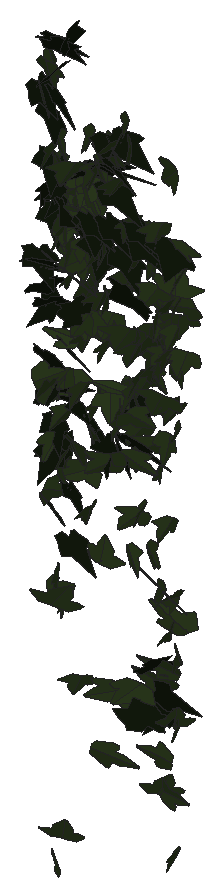
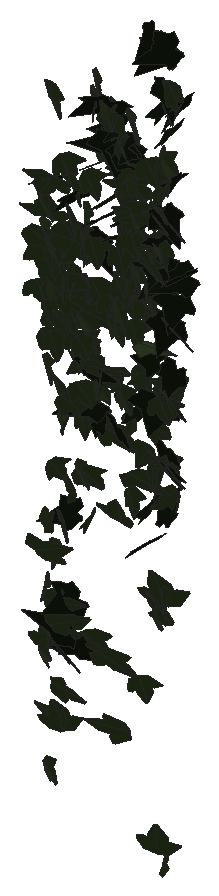
# SketchUp Ruby script. Lengths in millimetres.
U = 1.mm
M = Sketchup.active_model
def pt(a) = Geom::Point3d.new(a.map { |v| v * U })
def face(e, loops, mat)
  f = e.add_face(loops[0].map { |a| pt(a) })
  loops[1..].each { |l| e.add_face(l.map { |a| pt(a) }).erase! }
  f.material = f.back_material = mat if mat
  f
end
# faces: each face lists its corners as indices into pts; further lists are holes
def faces(e, pts, list, mat = nil) = list.each { |f| face(e, (f[0].is_a?(Array) ? f : [f]).map { |l| l.map { |i| pts[i] } }, mat) }
# xy, xz, yz: faces in a plane at the given z, y or x. An outline is a flat list of corners, or four numbers for a rectangle; further outlines are holes
def ring(l) = l.size == 4 ? [[l[0], l[1]], [l[2], l[1]], [l[2], l[3]], [l[0], l[3]]] : l.each_slice(2).to_a
def flat(e, list, mat, &to3) = list.each { |f| face(e, (f[0].is_a?(Array) ? f : [f]).map { |l| ring(l).map { |u, v| to3.(u, v) } }, mat) }
def xy(e, z, list, mat = nil) = flat(e, list, mat) { |x, y| [x, y, z] }
def xz(e, y, list, mat = nil) = flat(e, list, mat) { |x, z| [x, y, z] }
def yz(e, x, list, mat = nil) = flat(e, list, mat) { |y, z| [x, y, z] }
def lines(e, pts, list) = list.each { |a, b| e.add_line(pt(pts[a]), pt(pts[b])) }
# prism: a flat outline (further loops are holes) pulled along v
def prism(e, loops, v, mat = nil)
  f = face(e, loops, mat); d = Geom::Vector3d.new(v.map { |x| x * U })
  f.pushpull(f.normal.samedirection?(d) ? d.length : -d.length)
end
def box(e, o, s, mat = nil) = prism(e, [[o, [o[0] + s[0], o[1], o[2]], [o[0] + s[0], o[1] + s[1], o[2]], [o[0], o[1] + s[1], o[2]]]], [0, 0, s[2]], mat)
def at(x, y, z, deg = 0) = Geom::Transformation.translation(pt([x, y, z])) * Geom::Transformation.rotation(ORIGIN, Z_AXIS, deg.degrees)
def axes(o, x, y, z) = Geom::Transformation.new([*x, 0, *y, 0, *z, 0, *pt(o).to_a, 1])
def part(name) = M.definitions.add(name)
# library, detail: a bought-in or finely detailed component or shape, given as its bounding box
def library(name, o, s) = part(name).tap { |d| box(d.entities, o, s) }
def detail(e, o, s) = box(e.add_group.entities, o, s)
def put(e, d, t, mat = nil) = e.add_instance(d, t).tap { |i| i.material = mat if mat }
def group(e, t, mat = nil) = e.add_group.tap { |g| g.transformation = t; g.material = mat if mat }.entities
root = M.entities
M.materials.add("efeu1").color = [18, 25, 13]
M.materials.add("efeu2").color = [43, 57, 29]
c1 = part("ivyleaf_9")
p = [[39.1,54.8,31.7],[34.5,51.8,30.2],[-5.3,25.2,17.3],[-17.9,28.3,20.9],[-21.6,21.7,17],[-20.2,4.3,5.3],
  [-22.9,-0.3,2.5],[-17.1,-4,-0.6],[-2,-2.1,-1.2],[-0.7,-15.4,-10.1],[16.6,-22.3,-16.7],[21.1,-15.1,-12.5],
  [32.7,-10.7,-11],[46.1,-1.8,-6.6],[30.8,11.2,3.8]]
faces(c1.entities,p,[[0,1,2,3,4,5,6,7,8,9,10,11,12,13,14]],"efeu1")
c2 = part("ivyleaf_10")
p = [[0,12.8,-0.8],[-1.5,51.3,-10.9],[-4.9,51,-11.6],[-13.6,26.5,-7.3],[-13.2,15.9,-4.6],[-21.1,19.3,-7.2],
  [-29.5,16.3,-8.3],[-29.2,8.3,-6.2],[-19.7,-9.8,0.5],[-7.6,-13,4],[1,-12.2,5.8],[-0.4,51.1,-11.1],
  [-1.5,51.1,-10.9],[1,-12.4,5.9],[16.9,-12.4,3.5],[35.1,9.1,-5.1],[35,12.9,-6.1],[20.5,16.4,-4.9],
  [15.8,15,-3.8],[15.3,27.6,-7.1],[12.8,31.3,-7.8]]
faces(c2.entities,p,[[0,1,2,3,4,5,6,7,8,9,10],[11,12,0,13,14,15,16,17,18,19,20]],"efeu2")
put(root,c1,axes([810.5,996.7,1201],[0.11506,-0.81585,-0.18626],[0.13224,0.19777,-0.81138],[1.01235,0.06689,0.12716]))
put(root,c1,axes([829,1016.4,1320.9],[0.0026,0.65958,-0.47998],[0.00539,-0.47998,-0.65957],[-0.99518,-0.00087,-0.00482]))
put(root,c1,axes([825,987,1153.9],[0.42912,0.77528,0.01543],[-0.03301,0.0292,-0.85055],[-0.94545,0.35086,0.0367]))
put(root,c1,axes([834.5,1004,1112.6],[-0.90751,0.29825,-0.1157],[0.10865,-0.08822,-0.79997],[-0.37486,-0.74762,0.04824]))
put(root,c2,axes([829.4,1024.7,975],[-0.67201,-0.58372,0.16905],[-0.05048,-0.18053,-0.67875],[1.1555,-0.34737,0.06866]))
put(root,c1,axes([810.7,979.3,1192.1],[0.97056,0.14562,0.3072],[0.30233,0.2868,-0.77769],[-0.28395,0.80312,0.22202]))
put(root,c2,axes([813.2,1019.4,1543.2],[0.66337,-0.38918,0.43163],[0.57841,-0.04483,-0.63768],[0.41008,0.69279,0.20121]))
put(root,c1,axes([822.5,996.2,1025],[0.90634,0.10167,-0.35465],[-0.43015,-0.03911,-0.74979],[-0.13252,0.82229,0.00819]))
put(root,c1,axes([823.6,1004.6,1115],[0.72058,0.53904,-0.10921],[-0.11452,-0.0591,-0.7994],[-0.66114,0.59774,0.01944]))
put(root,c2,axes([827.9,999.2,1539.6],[-0.93809,0.19423,-0.00204],[0.00246,-0.00033,-0.79308],[-0.23696,-0.76893,-0.00017]))
put(root,c1,axes([819.5,985,1509.9],[0.38084,-0.64426,-0.50578],[-0.29332,0.44535,-0.71567],[0.95525,0.3936,-0.01811]))
put(root,c1,axes([840.7,1016.9,1320.5],[-0.80703,0.43923,0.04747],[-0.05481,0.01816,-0.79398],[-0.53618,-0.66295,0.00971]))
put(root,c2,axes([824.1,1024.8,623.6],[0.38639,-0.70982,0.08083],[0.19588,-0.01543,-0.76463],[0.84928,0.3265,0.13958]))
put(root,c2,axes([829.5,1012,866.3],[0.65073,0.43394,-0.30362],[-0.28178,-0.19718,-0.68757],[-0.58144,0.58121,-0.00658]))
put(root,c2,axes([824.3,989.7,1500.2],[-0.30724,0.76906,-0.17946],[0.02498,-0.18053,-0.78547],[-1.50279,-0.16023,0.02363]))
put(root,c2,axes([830,1011.9,1374],[-0.74422,0.53273,0.01084],[-0.0148,0.00259,-0.80987],[-0.6499,-0.61011,0.00602]))
put(root,c1,axes([831.1,985.7,952],[-0.64911,0.64885,0.05088],[0.02724,-0.04748,0.839],[0.79356,0.53237,0.01282]))
put(root,c1,axes([822,1021.8,893.4],[-0.5232,-0.16914,-0.62901],[0.75846,0.1184,-0.4557],[0.23709,-0.75203,0.06972]))
put(root,c1,axes([834.2,1005.5,849.9],[-0.87825,-0.08211,-0.33222],[0.4085,-0.00923,-0.72328],[0.08621,-0.79279,0.04282]))
put(root,c2,axes([820.4,1017.4,978.1],[0.70979,-0.24084,0.46021],[0.54301,-0.12506,-0.62813],[0.32666,0.73119,0.04415]))
put(root,c1,axes([842.1,990.6,1533.2],[-0.08532,0.8345,0.0914],[-0.02687,0.08986,-0.8373],[-1.02382,-0.0719,0.01435]))
put(root,c1,axes([829.3,1008.1,1370.5],[-0.10934,-0.82441,0.06829],[-0.02446,-0.0665,-0.82917],[1.00893,-0.09096,-0.0127]))
put(root,c1,axes([853.1,1011.4,860.7],[-0.85867,0.37249,0.21429],[-0.22636,0.10751,-0.79628],[-0.47289,-0.72783,-0.00795]))
put(root,c1,axes([844.2,1018.4,1307.9],[-0.86231,0.26897,-0.29214],[0.30251,-0.16693,-0.75361],[-0.37841,-0.74637,0.06327]))
put(root,c2,axes([819,1026.4,587],[0.82164,-0.31501,-0.50248],[0.7449,-0.3156,0.53413],[-0.84799,-0.58245,-0.01767]))
put(root,c2,axes([839.3,1020.9,159],[-1.16169,-0.28412,0.00304],[0.02764,-0.024,0.6727],[-0.54007,0.60992,0.02788]))
put(root,c2,axes([838.7,998.5,1399.6],[0.28935,-0.66536,0.39424],[0.15419,-0.38587,-0.68248],[1.46381,0.17217,-0.00604]))
put(root,c2,axes([841.8,1009.1,1256.9],[0.93948,-0.49893,-0.30782],[-0.14501,0.3444,-0.6804],[1.10628,0.46884,0.17223]))
put(root,c2,axes([846.7,1003.9,826.1],[-0.28859,0.32204,0.73224],[-0.49041,0.61231,-0.39915],[-0.84374,-0.46605,-0.01845]))
put(root,c1,axes([835.5,1019.9,1271.6],[-0.44811,-0.67676,-0.18819],[0.16019,0.14248,-0.76863],[0.84187,-0.38734,0.04608]))
put(root,c2,axes([837.7,1011.4,1365.1],[-0.22319,0.76666,0.10713],[-0.00851,0.10844,-0.78797],[-0.94437,-0.18217,-0.01822]))
put(root,c2,axes([842,1003.2,111.6],[-0.55913,0.52209,0.12956],[0.09511,-0.10394,0.69464],[0.64934,0.46478,0.00981]))
put(root,c2,axes([837.8,975.5,965],[0.10638,-0.45049,0.76235],[-0.04277,0.76368,0.45529],[-1.07946,-0.07465,0.05709]))
put(root,c1,axes([839.5,999.9,747.9],[0.61069,-0.60501,0.06345],[-0.02629,0.06448,0.78486],[-0.74169,-0.50043,0.02442]))
put(root,c1,axes([830.2,1003.1,1454],[0.09681,-0.75562,0.34801],[0.13592,-0.33679,-0.75665],[1.00578,0.11824,0.06876]))
put(root,c2,axes([836.1,988.1,790.7],[-0.17922,-0.3112,-0.73197],[0.44016,0.6373,-0.34335],[0.86479,-0.38886,0.02307]))
put(root,c2,axes([833,995.9,976.6],[0.23446,0.47738,0.64728],[0.26902,0.60873,-0.51442],[-0.94362,0.29216,0.01417]))
put(root,c2,axes([828.7,979,989.3],[0.21438,0.13816,-0.8179],[0.76135,0.52876,0.22339],[0.66667,-0.64827,0.00789]))
put(root,c2,axes([846.1,1017.2,920.3],[-0.11888,-0.46927,0.50324],[0.08472,-0.50701,-0.46726],[1.30683,-0.00982,0.07607]))
put(root,c2,axes([843,1005.7,1416.2],[-0.37776,0.74695,0.02492],[-0.00674,0.02469,-0.80857],[-0.91176,-0.30966,-0.00435]))
put(root,c2,axes([842.6,1019,1321.3],[0.82884,-0.38508,0.03991],[0.06123,0.00769,-0.78029],[0.46832,0.68051,0.0314]))
put(root,c2,axes([848.5,1010.4,1251.7],[0.38343,-0.68889,0.26418],[0.10778,-0.25861,-0.71754],[1.40006,0.20857,-0.01711]))
put(root,c1,axes([849.5,1006.9,962.3],[0.70695,0.6692,0.00724],[0.0069,0.00627,-0.76538],[-1.27368,0.37147,-0.00013]))
put(root,c2,axes([870.3,1010.8,1058.5],[-0.01452,0.91215,0.07957],[-1.07438,-0.03318,0.24871],[0.30578,-0.07329,0.87767]))
put(root,c2,axes([837.8,1024.6,580.7],[0.23864,-0.16207,0.709],[0.72435,-0.59846,-0.20411],[1.17951,0.40031,-0.0181]))
put(root,c2,axes([852.2,1007.8,1264.7],[0.29034,0.71243,-0.24275],[-0.36565,-0.20262,-0.7154],[-1.38499,0.20284,0.13798]))
put(root,c1,axes([843.5,987.1,1186.7],[0.98595,0.32085,0.07328],[-0.10674,0.39675,-0.77225],[-0.38707,0.70787,0.39962]))
put(root,c2,axes([853.6,1013.3,850.4],[0.05824,-0.76718,-0.28533],[0.04288,0.28747,-0.76706],[0.99767,0.03243,0.04963]))
put(root,c2,axes([858.1,1019.2,1169.1],[0.10324,-0.72495,-0.16649],[-0.01858,0.16623,-0.72697],[1.41552,0.05506,0.0026]))
put(root,c2,axes([850.4,1009.2,1257.6],[0.44957,0.71549,-0.13948],[-0.07134,-0.13451,-0.75345],[-1.38553,0.23909,-0.00647]))
put(root,c1,axes([839.5,981.5,1600.2],[0.98244,0.05569,0.29584],[0.35171,0.1006,-0.80366],[-0.10574,0.85198,0.07556]))
put(root,c2,axes([850.8,987,594.1],[-1.28446,-0.37921,0.22381],[0.37788,0.10352,0.77411],[-0.74801,0.70346,0.00674]))
put(root,c1,axes([843.4,993.7,1498.5],[0.62538,-0.65051,0.08874],[0.04965,-0.08088,-0.82802],[0.79944,0.51391,-0.01799]))
put(root,c1,axes([845.5,1028.6,779.7],[0.46995,-0.67238,0.08197],[0.05356,-0.06932,-0.7749],[0.82464,0.38768,0.00361]))
put(root,c1,axes([852.3,980.9,1596.9],[1.01157,0.26779,0.07465],[0.08886,0.01735,-0.87131],[-0.32731,0.83233,-0.00585]))
put(root,c1,axes([844.5,1013.9,1041.4],[0.61009,-0.48001,0.43659],[0.39567,-0.29251,-0.69307],[0.68563,0.59592,0.01148]))
put(root,c2,axes([881.3,1025.1,824.3],[0.84323,0.17571,-0.55178],[-1.00277,-0.16596,-0.47591],[-0.4573,0.68791,0.02613]))
put(root,c2,axes([872.8,1022.1,450.5],[-0.6644,-0.54002,0.09315],[-0.07201,-0.08643,-0.64286],[1.04045,-0.35082,0.01499]))
put(root,c2,axes([878.2,993.8,1378.6],[-0.63834,-0.69105,0.19205],[-0.09949,-0.18789,-0.7674],[1.36143,-0.33775,0.03397]))
put(root,c2,axes([871.3,1011.7,870.9],[-1.09488,0.35322,-0.00911],[0.02595,0.0048,-0.67498],[-0.67198,-0.57534,-0.01122]))
put(root,c2,axes([885.2,998.3,1212],[1.04737,-0.39006,-0.3983],[-0.59891,0.24463,-0.67436],[0.8758,0.63376,0.01516]))
put(root,c1,axes([847.7,991.3,1196.9],[0.77809,-0.53526,0.38014],[0.56383,-0.24923,-0.66954],[1.11503,0.49954,0.07329]))
put(root,c1,axes([865.9,1005.4,1287.6],[0.66944,-0.41941,-0.54577],[0.63238,-0.4333,0.54712],[-1.14724,-0.48357,-0.01689]))
put(root,c1,axes([882.2,979.1,1615],[-0.05789,0.21163,-0.80134],[-0.92243,0.64594,0.18899],[1.27957,0.47522,0.09999]))
put(root,c1,axes([864.8,1007.3,702.6],[0.38826,-0.66947,-0.30407],[-0.12032,0.29841,-0.69944],[1.39422,0.21219,0.02431]))
put(root,c2,axes([873.1,998.7,1235.5],[0.32351,-0.54115,0.49831],[0.45034,-0.44404,-0.56293],[1.32565,0.28291,0.06963]))
put(root,c1,axes([905,980.7,1129],[-0.73145,0.61801,0.33207],[-0.36453,0.27183,-0.72756],[-1.28451,-0.42906,0.01737]))
put(root,c2,axes([878.7,1001,1000.2],[0.31694,0.742,-0.15425],[-0.10042,-0.1462,-0.76022],[-1.43887,0.17364,0.01908]))
put(root,c2,axes([890.2,1014.8,1184.4],[0.47793,-0.6677,-0.2251],[-0.09366,0.22177,-0.71271],[1.33776,0.25407,0.03052]))
put(root,c1,axes([884.6,1020.2,929.1],[0.68139,-0.64465,-0.23053],[0.20534,-0.20377,0.73738],[-1.2867,-0.3739,-0.0044]))
put(root,c2,axes([875,1004.2,1300.6],[-0.71988,-0.2227,-0.63961],[1.04117,0.33142,-0.43892],[0.75989,-0.66508,-0.00455]))
put(root,c2,axes([897.7,1006,1290],[0.2494,-0.75965,0.0594],[0.00385,-0.05993,-0.77082],[1.45017,0.1308,-0.00817]))
put(root,c2,axes([884.2,1004.7,1291.2],[1.2428,0.3271,0.26082],[0.32214,0.23557,-0.71923],[-0.72813,0.66253,0.12697]))
put(root,c2,axes([900.7,1000.6,1345.4],[-0.1602,-0.76029,0.17337],[0.00501,-0.17465,-0.76463],[1.48411,-0.08148,0.02129]))
put(root,c2,axes([900.2,1009.4,917.2],[-0.80892,0.51446,0.15576],[-0.22671,0.10349,-0.66685],[-0.99758,-0.44069,0.02524]))
put(root,c2,axes([899.8,993.6,992],[-0.03057,-0.70344,0.30525],[0.06398,-0.30567,-0.70264],[1.458,-0.00134,0.03724]))
put(root,c2,axes([901.1,1004,1081.8],[-0.22628,-0.71558,-0.0452],[0.0173,0.04431,-0.72539],[1.3645,-0.11923,0.0017]))
put(root,c2,axes([904.4,1004.9,1243.6],[-0.81794,-0.6068,0.16225],[0.05903,-0.21686,-0.72886],[1.19397,-0.40497,0.14719]))
put(root,c2,axes([905.2,1005.2,773.9],[-0.08207,-0.71516,-0.12819],[0.03532,0.12729,-0.71637],[1.38233,-0.04571,0.01069]))
put(root,c2,axes([905.1,989.4,1119.7],[1.11794,-0.51934,-0.13296],[-0.17581,0.09624,-0.78399],[1.00503,0.59452,0.01076]))
put(root,c2,axes([903.9,1013.4,1158.3],[0.07518,-0.63707,-0.38176],[0.24876,0.3823,-0.62444],[1.39144,-0.03392,0.13226]))
put(root,c2,axes([905.8,998.3,1176.3],[-0.24438,-0.62417,-0.3879],[0.26023,0.36661,-0.63517],[1.37421,-0.18042,0.0513]))
put(root,c2,axes([912.3,1017.8,959.3],[0.0663,-0.6922,0.12796],[0.04246,-0.12697,-0.6929],[1.33905,0.0383,0.01563]))
put(root,c2,axes([909.3,996,1360],[1.07492,0.5157,-0.19304],[-0.24234,-0.14672,-0.7645],[-1.01959,0.57856,-0.0218]))
put(root,c2,axes([903.2,997.1,1121.1],[1.42153,-0.05179,0.1256],[0.23884,-0.00583,-0.74871],[0.09904,0.75738,0.00283]))
put(root,c1,axes([928.1,995.2,1391.5],[-0.43505,0.58321,-0.48952],[-0.03409,-0.51508,-0.6053],[-1.44873,-0.16301,0.16124]))
put(root,c2,axes([917.3,1023,1119.5],[0.05485,-0.73569,-0.00337],[-0.00014,0.00337,-0.73625],[1.40017,0.02882,0.00006]))
put(root,c2,axes([917.6,991.1,1450.9],[0.592,-0.7327,-0.08513],[-0.03991,0.08356,-0.79589],[1.40329,0.31148,0.01328]))
put(root,c2,axes([910.5,1000,1341.6],[-0.02355,0.78489,-0.00492],[0.01202,-0.00482,-0.78496],[-1.49379,-0.01241,-0.00624]))
put(root,c2,axes([916.1,1019.4,981.5],[-0.14034,0.69346,0.04447],[-0.19292,0.03351,-0.69058],[-1.30836,-0.07932,0.09706]))
put(root,c2,axes([904.6,1001.6,1333.9],[1.25995,0.34794,0.23836],[0.29577,0.21117,-0.73986],[-0.7462,0.67119,0.10921]))
put(root,c2,axes([909.8,999,1363.9],[0.68312,0.62564,0.32056],[0.02447,0.35402,-0.70535],[-1.33769,0.32597,0.1508]))
put(root,c2,axes([921.7,1013.9,1154.8],[-0.31265,-0.72316,0.04762],[0.01424,-0.05052,-0.74135],[1.37922,-0.16341,0.01845]))
put(root,c1,axes([909.2,1007.6,1277.7],[-0.14897,-0.6945,0.32015],[0.01532,-0.32255,-0.69775],[1.45537,-0.06769,0.04012]))
put(root,c2,axes([924.3,1010.6,1208.9],[-0.52476,-0.70069,-0.03012],[0.01103,0.03008,-0.75296],[1.33473,-0.27573,-0.00562]))
put(root,c2,axes([930.1,994.4,1396.6],[-0.09839,-0.69287,0.38897],[0.04318,-0.39092,-0.69333],[1.51164,-0.03393,0.04512]))
put(root,c1,axes([913.3,992.4,1301.4],[0.61665,-0.62124,-0.31863],[-0.16058,0.31385,-0.69772],[1.31904,0.32864,0.06402]))
put(root,c2,axes([931.3,992.5,1245.1],[0.06641,-0.71905,-0.24535],[0.09756,0.24728,-0.71741],[1.44268,0.01638,0.05981]))
put(root,c1,axes([925.9,1010,1242.4],[-0.39553,-0.71014,0.17606],[-0.08603,-0.17021,-0.73991],[1.3898,-0.21264,0.0043]))
put(root,c2,axes([948.5,1003,872.5],[-0.76387,-0.3555,0.47741],[-0.59079,-0.36629,-0.53373],[0.9666,-0.50482,0.05106]))
put(root,c2,axes([930.3,994.8,1398.4],[0.4559,-0.63784,0.41313],[0.27504,-0.38703,-0.68134],[1.41994,0.27976,-0.00067]))
put(root,c2,axes([934.1,1008.2,1159.2],[0.41711,-0.61722,-0.35918],[0.08501,0.38683,-0.63748],[1.35646,0.16555,0.1504]))
put(root,c1,axes([923.6,1018.4,896.6],[-0.72065,0.06007,-0.67401],[1.24659,-0.16141,-0.38236],[-0.3234,-0.75605,0.02808]))
put(root,c2,axes([938.4,1014.9,1120.3],[-0.7931,-0.55756,0.23996],[0.04881,-0.30698,-0.66874],[1.15421,-0.37013,0.19317]))
put(root,c2,axes([938.5,1009.1,1077.6],[0.05664,-0.74264,0.11593],[0.00037,-0.11601,-0.74323],[1.43051,0.02943,-0.0044]))
put(root,c2,axes([931.5,994.5,1403.3],[-0.32578,0.77991,-0.00669],[0.01069,-0.00562,-0.79846],[-1.48434,-0.17122,-0.00428]))
put(root,c2,axes([954.5,1009.3,463.6],[0.97687,0.03697,-0.5499],[-1.04616,-0.0203,-0.51444],[-0.07626,0.75195,0.01315]))
put(root,c1,axes([942.8,993.9,1400.2],[0.60902,0.72404,-0.0972],[-0.06022,-0.09228,-0.79155],[-1.38904,0.32145,-0.0083]))
put(root,c2,axes([949.8,1005.9,1104.7],[0.51791,-0.65517,-0.26788],[-0.15303,0.25652,-0.70908],[1.3384,0.28285,0.02258]))
put(root,c2,axes([951.8,979.7,1256.3],[0.21549,-0.55693,-0.58004],[-0.17041,0.57339,-0.56802],[1.5209,0.14316,0.01854]))
put(root,c2,axes([921.6,1013.4,341.6],[-0.22988,0.02245,-0.72965],[1.36535,-0.13318,-0.12285],[-0.25704,-0.72749,-0.00003]))
put(root,c2,axes([951.8,990.7,1435.6],[-1.21902,0.47934,0.07627],[-0.12007,0.04299,-0.80001],[-0.91592,-0.6436,0.00337]))
put(root,c2,axes([972.8,1022.7,990.7],[0.0426,0.33325,0.63084],[-1.14534,-0.3302,0.19579],[0.72936,-0.53799,0.2706]))
put(root,c2,axes([975.3,1016.9,1084.1],[0.37374,0.02791,-0.7104],[-1.33251,0.13556,-0.18821],[0.23494,0.72446,0.06258]))
put(root,c2,axes([946.5,984.5,707],[1.29784,-0.19023,0.01699],[-0.02649,0.01334,0.7079],[-0.36253,-0.682,0.0091]))
put(root,c2,axes([948.2,1002.3,983.3],[0.97296,0.47958,-0.03422],[-0.05059,-0.02167,-0.70096],[-0.91366,0.51191,0.00238]))
put(root,c1,axes([925.6,995.2,1396.8],[1.28473,-0.14654,0.39692],[0.80197,0.16539,-0.65558],[0.07268,0.76542,0.21765]))
put(root,c1,axes([945.4,999.7,1300.6],[0.55663,-0.67636,-0.23949],[-0.127,0.23186,-0.73631],[1.35965,0.29856,0.02927]))
put(root,c2,axes([958,989.1,1452.3],[-0.56845,0.74738,-0.07122],[0.0374,-0.06884,-0.80482],[-1.42837,-0.29924,0.00727]))
put(root,c2,axes([968.3,988.4,1454.7],[-0.05363,-0.80038,-0.11798],[-0.03768,0.11869,-0.80053],[1.53929,-0.02498,-0.02371]))
put(root,c2,axes([963.8,1004.7,969.3],[0.14897,-0.57667,-0.49339],[0.16962,0.49955,-0.56974],[1.4344,0.00082,0.11861]))
put(root,c2,axes([969.9,994.1,1382.3],[-0.18553,-0.77423,0.14032],[-0.06819,-0.13688,-0.78013],[1.49596,-0.10226,-0.01816]))
put(root,c1,axes([943.7,992.3,1424.4],[0.76687,-0.67919,0.14319],[0.14514,-0.12125,-0.78971],[1.31306,0.41008,0.00366]))
put(root,c2,axes([967.5,1008.4,950.6],[0.08635,-0.64459,0.28294],[0.09431,-0.2799,-0.6456],[1.33643,0.0614,0.02728]))
put(root,c2,axes([974.9,1016.4,1210.9],[-0.50743,-0.69959,0.04964],[0.02259,-0.0576,-0.74801],[1.33463,-0.26501,0.03153]))
put(root,c1,axes([955.2,996.8,1365.2],[0.368,-0.71103,-0.28018],[0.12761,0.30368,-0.72439],[1.4489,0.15385,0.13496]))
put(root,c1,axes([999.7,1007.1,973.1],[-0.31562,0.18295,0.73012],[-0.84291,0.58079,-0.24613],[-1.15828,-0.47251,-0.01984]))
put(root,c1,axes([963.8,1014.5,876.2],[-0.09934,-0.02203,0.75998],[0.02939,-0.76165,-0.02102],[1.44671,0.01396,0.05261]))
put(root,c2,axes([990.8,993.7,1121.6],[-1.03825,-0.51842,0.24353],[-0.27778,-0.19939,-0.7514],[1.05411,-0.56316,0.04185]))
put(root,c2,axes([977,1017.9,714.2],[-0.17544,0.7292,-0.07445],[0.01529,-0.07403,-0.73501],[-1.39495,-0.09252,0.00131]))
put(root,c2,axes([993,1016.2,787.9],[-0.65777,-0.38296,0.42339],[-0.30333,-0.41053,-0.50143],[1.04333,-0.36079,0.12115]))
put(root,c1,axes([965.1,988.6,1462.3],[0.01125,-0.44392,-0.67778],[0.42251,0.65274,-0.42559],[1.48299,-0.1826,0.1264]))
put(root,c2,axes([996.4,1004.9,484.2],[1.05633,0.32084,-0.42443],[-0.73127,-0.18256,-0.64045],[-0.70044,0.67444,0.02855]))
put(root,c2,axes([996.2,1020.8,942.8],[-0.62532,-0.58881,0.2804],[-0.17213,-0.26981,-0.67254],[1.22922,-0.33732,0.04847]))
put(root,c2,axes([991.3,985.5,1497.4],[0.51819,-0.72391,-0.265],[-0.01694,0.27807,-0.76877],[1.46706,0.25891,0.08472]))
put(root,c1,axes([977.7,1003.8,1249.4],[0.03746,-0.76216,-0.05621],[-0.00568,0.05615,-0.76241],[1.45447,0.01985,-0.00153]))
put(root,c2,axes([992.5,1017.2,1211.9],[0.2731,-0.65581,-0.33627],[0.02673,0.34496,-0.66675],[1.4024,0.12114,0.07819]))
put(root,c1,axes([1010.6,978.3,1199.7],[0.47829,0.19547,-0.76499],[-1.47879,-0.08144,-0.27606],[-0.26704,0.80108,0.1586]))
put(root,c2,axes([993.3,1016.5,1215.9],[0.23886,-0.71483,-0.19602],[0.01417,0.20002,-0.72463],[1.41062,0.11903,0.04047]))
put(root,c2,axes([997.1,1019.7,1025.3],[-0.35238,-0.64663,0.20315],[-0.10395,-0.19567,-0.67261],[1.28577,-0.19304,0.0013]))
put(root,c2,axes([987.9,1014.6,1003.3],[-0.33734,0.70809,0.03896],[-0.01272,0.03848,-0.72993],[-1.34961,-0.17735,-0.00286]))
put(root,c2,axes([994.1,1020.1,890.7],[-0.1777,-0.67371,-0.07354],[0.03578,0.07163,-0.6801],[1.28933,-0.09484,0.00874]))
put(root,c2,axes([996.1,1000.7,1318.7],[-0.16887,-0.75427,0.18352],[0.03882,-0.18692,-0.75836],[1.47689,-0.08133,0.04092]))
put(root,c2,axes([994.3,1025.3,797.5],[0.40443,-0.65227,0.15038],[0.07317,-0.14562,-0.68596],[1.27186,0.21579,-0.00836]))
put(root,c1,axes([973.5,1008.5,919.6],[1.46702,-0.16365,0.08586],[0.15966,-0.0183,-0.788],[0.3134,0.77537,-0.00048]))
put(root,c2,axes([1000.3,1001.8,1260.1],[0.26067,-0.67875,-0.32838],[0.05847,0.3385,-0.68686],[1.43384,0.10959,0.08771]))
put(root,c2,axes([997.4,997.4,1017.9],[0.10461,-0.55075,0.46875],[0.25001,-0.45468,-0.54962],[1.35354,0.12655,0.06529]))
put(root,c2,axes([1006.3,1018.2,1030.3],[-0.64904,-0.60164,0.13266],[-0.0969,-0.12359,-0.69138],[1.16854,-0.34442,0.01635]))
put(root,c2,axes([1001.6,981.5,1461.6],[0.52325,-0.71871,-0.2534],[0.13728,0.29272,-0.75197],[1.44387,0.23262,0.16333]))
put(root,c2,axes([1016.2,1029.5,916.5],[-0.58921,-0.43686,0.45969],[-0.46162,-0.39108,-0.535],[1.11516,-0.39271,0.02142]))
put(root,c2,axes([1008.5,990.9,1100.7],[-0.43408,-0.69401,0.0999],[-0.04244,-0.09782,-0.73047],[1.33378,-0.22898,0.00927]))
put(root,c2,axes([988.6,993.4,900.3],[-0.90672,-0.18975,-0.51841],[0.95782,0.13214,-0.51087],[0.4318,-0.69156,0.04463]))
put(root,c2,axes([1012,986.9,1118.3],[0.38761,-0.64066,-0.42388],[-0.13095,0.42155,-0.67019],[1.45614,0.20844,0.05256]))
put(root,c2,axes([1018.8,1026.2,1099.8],[-0.34545,-0.41509,0.5609],[-0.22745,-0.55251,-0.44755],[1.3084,-0.20564,0.07029]))
put(root,c2,axes([1003.4,986.5,982.7],[-0.65582,-0.44133,-0.53872],[0.70196,0.3942,-0.55885],[1.12428,-0.50356,0.03467]))
put(root,c2,axes([1012.5,994.6,1051.7],[0.40388,-0.65109,0.3794],[0.18762,-0.36678,-0.68457],[1.42186,0.23334,-0.01744]))
put(root,c1,axes([1003.3,998.4,1315.2],[0.48886,-0.70449,-0.20401],[-0.04832,0.20749,-0.74847],[1.39504,0.25406,0.04556]))
put(root,c2,axes([1042.6,1020.9,497.3],[-0.74057,-0.02553,-0.61373],[-1.15906,-0.07879,0.3894],[-0.15258,0.72241,0.02078]))
put(root,c2,axes([1020.5,1020.3,1132.8],[-0.66257,-0.62884,-0.16639],[0.20396,0.13069,-0.71816],[1.22108,-0.36304,0.02967]))
put(root,c1,axes([1028.4,994.6,435.1],[-1.29214,-0.21061,0.3147],[0.58598,0.06907,0.71047],[-0.41955,0.74513,0.02309]))
put(root,c2,axes([1020.5,1019,1194.9],[-1.37244,-0.02035,-0.16316],[0.31277,-0.06539,-0.71817],[0.01016,-0.73645,0.06828]))
put(root,c1,axes([1010.9,1004.6,1287.7],[0.33449,-0.63052,-0.48216],[-0.16183,0.47604,-0.65351],[1.50197,0.19171,0.03696]))
put(root,c2,axes([1024.5,1012.8,1251.9],[0.74996,-0.64188,-0.09922],[0.02491,0.12387,-0.74941],[1.23588,0.38701,0.07531]))
put(root,c2,axes([1029.9,1003,1308.3],[0.85674,-0.63597,-0.24936],[-0.1665,0.2425,-0.77641],[1.28938,0.45389,0.06543]))
put(root,c2,axes([1023.9,1034.4,876],[-0.12537,0.04333,-0.70255],[-0.0442,-0.70537,-0.04133],[-1.33891,0.01923,0.06715]))
put(root,c2,axes([1026.1,1014.1,1119.2],[-0.8112,0.61962,0.01152],[-0.01505,0.00855,-0.75207],[-1.17938,-0.4263,0.00167]))
put(root,c2,axes([1050.9,1011.1,373.5],[0.00403,0.06646,0.66374],[-1.26774,0.03558,-0.00144],[-0.06765,-0.66279,0.06648]))
put(root,c2,axes([1028.9,1013.3,1127.6],[-0.00911,-0.64637,-0.35972],[0.17592,0.35638,-0.6416],[1.3968,-0.0491,0.07846]))
put(root,c2,axes([1033.2,1005.7,1069.8],[-0.09229,-0.71919,-0.11963],[0.04775,0.11817,-0.72062],[1.38674,-0.05193,0.01685]))
put(root,c2,axes([1040.2,1000.7,1211.6],[-0.87435,-0.51113,0.3166],[-0.18721,-0.32918,-0.67418],[1.12887,-0.45048,0.13341]))
put(root,c2,axes([1037.2,999,1081.4],[0.86433,-0.45244,-0.34408],[-0.20748,0.36291,-0.62109],[1.06173,0.43925,0.15874]))
put(root,c2,axes([1058.9,1014.1,530.6],[-0.31105,0.09841,-0.64148],[-1.22442,0.06241,0.17349],[0.16241,0.65902,0.07936]))
put(root,c1,axes([1025,996.1,536.4],[0.67921,0.4478,0.5238],[0.63424,0.40416,-0.57258],[-1.14799,0.48824,-0.00643]))
put(root,c2,axes([1021.3,1015.7,1056],[-0.53117,0.20552,-0.62921],[0.64183,-0.54344,-0.32709],[-1.08402,-0.42247,0.11465]))
put(root,c2,axes([1035.6,989.9,1130.1],[-0.06653,-0.55942,-0.56628],[0.24147,0.55567,-0.55677],[1.4956,-0.1146,0.0647]))
put(root,c2,axes([1038.5,1019.1,1152.4],[0.61791,-0.62627,-0.21445],[0.03107,0.24636,-0.69473],[1.25947,0.30118,0.12235]))
put(root,c2,axes([1025.8,1006.4,739.6],[-0.11278,0.06737,-0.75086],[0.53873,-0.69608,-0.0848],[-1.3298,-0.28771,0.02933]))
put(root,c2,axes([1039.4,1015,311.4],[-0.95341,-0.5107,0.08638],[0.12531,0.05641,0.71534],[-0.97778,0.50521,0.00744]))
put(root,c2,axes([1043,1006.2,1161.5],[-0.01869,0.65143,-0.34534],[-0.23999,-0.34176,-0.6411],[-1.38256,0.05052,0.11596]))
put(root,c1,axes([1052.8,1019,459.6],[-1.18493,0.34576,-0.33148],[0.54368,-0.16831,-0.71212],[-0.73174,-0.68496,0.00766]))
put(root,c2,axes([1045.9,1027.4,787.3],[-0.27566,-0.54371,0.37865],[0.11247,-0.39665,-0.54694],[1.25597,-0.08381,0.13209]))
put(root,c2,axes([1052.6,1000.3,679.1],[0.36919,-0.59324,-0.38705],[-0.23004,0.36769,-0.62415],[1.32834,0.22856,-0.00051]))
put(root,c1,axes([1024.5,999.9,696.4],[1.20395,-0.47981,0.03558],[0.0477,-0.02583,-0.79395],[0.91444,0.63306,-0.00543]))
put(root,c2,axes([1050.5,996.5,1328.6],[-0.44763,-0.71325,0.21046],[0.05865,-0.2299,-0.74467],[1.41411,-0.21624,0.09751]))
put(root,c2,axes([1059,1010.1,1102.6],[-0.62914,-0.51756,0.37757],[-0.22028,-0.36963,-0.60801],[1.19921,-0.33943,0.0864]))
put(root,c2,axes([1055.7,1018,1188.7],[0.0803,-0.74568,-0.04214],[-0.04236,0.04093,-0.74661],[1.42082,0.04336,-0.01988]))
put(root,c2,axes([1064.5,985.9,1032.4],[-1.31948,-0.20216,0.22649],[-0.39964,-0.08847,-0.72174],[0.41729,-0.72397,0.02495]))
put(root,c2,axes([1057.6,1014.5,1010.4],[-0.31218,-0.67863,-0.0397],[-0.00883,0.04195,-0.69802],[1.29374,-0.16347,-0.01434]))
put(root,c2,axes([1058.9,1022.9,1147.8],[-0.43247,-0.68618,0.13756],[0.00444,-0.14537,-0.72129],[1.33191,-0.22232,0.04707]))
put(root,c2,axes([1059.1,1012,1100.4],[-0.0121,-0.72143,0.06981],[0.02206,-0.0699,-0.72136],[1.37926,-0.00521,0.01215]))
put(root,c2,axes([1049.2,1016.6,940.7],[1.04992,-0.48064,0.25433],[0.34498,-0.17904,-0.73152],[0.97574,0.58048,-0.01503]))
put(root,c2,axes([1077.7,1018.3,617.6],[0.94187,0.17402,0.59062],[-1.09421,-0.14063,0.52317],[0.41945,-0.75761,0.03855]))
put(root,c1,axes([1029,1018.1,485.9],[0.64281,-0.11441,-0.67583],[1.28112,0.19748,0.30298],[0.24607,-0.72926,0.18807]))
put(root,c2,axes([1064.3,1020,1140.1],[-0.19806,-0.64422,0.33473],[0.21031,-0.34827,-0.63592],[1.36561,-0.0398,0.14648]))
put(root,c2,axes([1071.7,1014.5,1073.8],[0.75712,-0.38453,-0.4634],[-0.28397,0.47513,-0.52235],[1.11031,0.38373,0.1824]))
put(root,c2,axes([1069.5,1016.6,964.6],[0.28952,-0.65836,-0.1441],[-0.02036,0.14535,-0.67536],[1.2825,0.15093,0.02181]))
put(root,c2,axes([1072.7,1019.4,1163.9],[-1.11706,-0.44455,0.0232],[-0.03547,-0.01382,-0.73629],[0.84647,-0.58724,-0.00024]))
put(root,c2,axes([1092.8,1018.2,1191],[-0.6404,0.00305,0.66554],[-1.2578,-0.08967,-0.33372],[0.1497,-0.74036,0.04316]))
put(root,c2,axes([1074,1013,1009.5],[-0.1995,-0.62984,0.28599],[-0.059,-0.28469,-0.63833],[1.31518,-0.10831,0.01475]))
put(root,c2,axes([1072.5,1012.8,666.9],[-0.15303,-0.13007,-0.65889],[-0.3432,-0.63505,0.14737],[-1.23126,0.19318,0.04081]))
put(root,c2,axes([1047,1013.6,311],[-0.37416,0.05078,0.69356],[1.27181,-0.18571,0.20302],[0.36636,0.69656,0.00356]))
put(root,c2,axes([1073,992,617.2],[-0.07208,-0.5861,-0.39692],[0.02199,0.39692,-0.58721],[1.34701,-0.03784,-0.01166]))
put(root,c2,axes([1066.6,1029,441],[0.39598,-0.47597,0.46003],[0.33179,-0.4258,-0.5194],[1.21535,0.27132,-0.00809]))
put(root,c2,axes([1071,1011.8,564.5],[0.32319,-0.51788,-0.43212],[0.16181,0.45848,-0.51607],[1.27343,0.07318,0.17524]))
put(root,c2,axes([1073.2,1008.2,447],[-0.75342,-0.53806,-0.08489],[-0.06206,-0.08135,0.66764],[-1.03484,0.39661,0.02177]))
put(root,c2,axes([1076.5,1004.7,217.7],[0.2915,-0.63183,0.17339],[0.0731,-0.1691,-0.65012],[1.24481,0.15789,-0.00243]))
put(root,c2,axes([1078.3,1011.9,1206.7],[0.42822,-0.71379,-0.01859],[0.00815,0.02085,-0.74834],[1.35892,0.2248,0.01035]))
put(root,c1,axes([1073.5,1005.7,1291.9],[-0.59724,-0.67981,0.19343],[-0.00864,-0.2097,-0.74434],[1.34515,-0.30318,0.08111]))
put(root,c2,axes([1084.7,984.8,1443.9],[0.83615,-0.54122,-0.47949],[-0.33051,0.46566,-0.68473],[1.33586,0.45398,0.13071]))
put(root,c2,axes([1066,1009.1,1295],[1.31242,0.17764,0.2602],[0.44264,0.13536,-0.70878],[-0.40448,0.72451,0.06863]))
put(root,c2,axes([1077.2,1002.8,1225.3],[1.40877,0.21742,-0.00704],[0.00697,0.01251,0.7714],[0.41395,-0.74014,0.01097]))
put(root,c2,axes([1084.8,1018.6,1100.1],[-0.87164,-0.52435,0.20699],[0.05296,-0.2874,-0.66646],[1.07157,-0.41231,0.20131]))
put(root,c2,axes([1082.6,1009.3,1252.9],[0.48043,-0.71206,0.1365],[0.04453,-0.13646,-0.75513],[1.37916,0.25245,-0.02317]))
